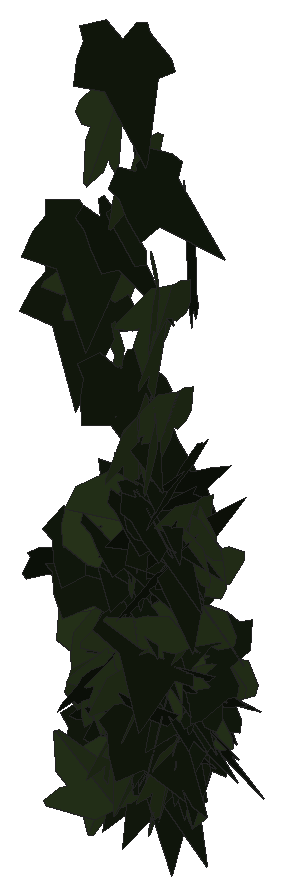
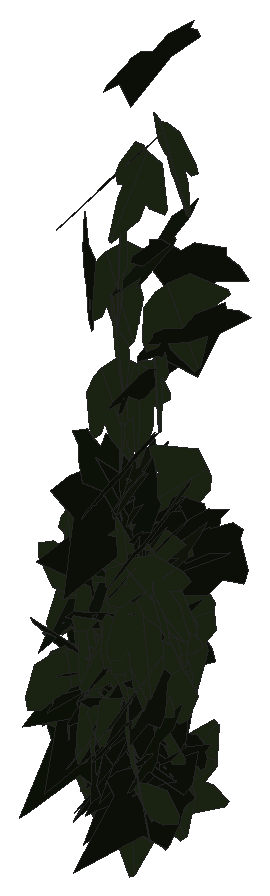
# SketchUp Ruby script. Lengths in inches.
U = 1.inch
M = Sketchup.active_model
def pt(a) = Geom::Point3d.new(a.map { |v| v * U })
def face(e, loops, mat)
  f = e.add_face(loops[0].map { |a| pt(a) })
  loops[1..].each { |l| e.add_face(l.map { |a| pt(a) }).erase! }
  f.material = f.back_material = mat if mat
  f
end
# faces: each face lists its corners as indices into pts; further lists are holes
def faces(e, pts, list, mat = nil) = list.each { |f| face(e, (f[0].is_a?(Array) ? f : [f]).map { |l| l.map { |i| pts[i] } }, mat) }
# xy, xz, yz: faces in a plane at the given z, y or x. An outline is a flat list of corners, or four numbers for a rectangle; further outlines are holes
def ring(l) = l.size == 4 ? [[l[0], l[1]], [l[2], l[1]], [l[2], l[3]], [l[0], l[3]]] : l.each_slice(2).to_a
def flat(e, list, mat, &to3) = list.each { |f| face(e, (f[0].is_a?(Array) ? f : [f]).map { |l| ring(l).map { |u, v| to3.(u, v) } }, mat) }
def xy(e, z, list, mat = nil) = flat(e, list, mat) { |x, y| [x, y, z] }
def xz(e, y, list, mat = nil) = flat(e, list, mat) { |x, z| [x, y, z] }
def yz(e, x, list, mat = nil) = flat(e, list, mat) { |y, z| [x, y, z] }
def lines(e, pts, list) = list.each { |a, b| e.add_line(pt(pts[a]), pt(pts[b])) }
# prism: a flat outline (further loops are holes) pulled along v
def prism(e, loops, v, mat = nil)
  f = face(e, loops, mat); d = Geom::Vector3d.new(v.map { |x| x * U })
  f.pushpull(f.normal.samedirection?(d) ? d.length : -d.length)
end
def box(e, o, s, mat = nil) = prism(e, [[o, [o[0] + s[0], o[1], o[2]], [o[0] + s[0], o[1] + s[1], o[2]], [o[0], o[1] + s[1], o[2]]]], [0, 0, s[2]], mat)
def at(x, y, z, deg = 0) = Geom::Transformation.translation(pt([x, y, z])) * Geom::Transformation.rotation(ORIGIN, Z_AXIS, deg.degrees)
def axes(o, x, y, z) = Geom::Transformation.new([*x, 0, *y, 0, *z, 0, *pt(o).to_a, 1])
def part(name) = M.definitions.add(name)
# library, detail: a bought-in or finely detailed component or shape, given as its bounding box
def library(name, o, s) = part(name).tap { |d| box(d.entities, o, s) }
def detail(e, o, s) = box(e.add_group.entities, o, s)
def put(e, d, t, mat = nil) = e.add_instance(d, t).tap { |i| i.material = mat if mat }
def group(e, t, mat = nil) = e.add_group.tap { |g| g.transformation = t; g.material = mat if mat }.entities
root = M.entities
M.materials.add("efeu1").color = [18, 25, 13]
M.materials.add("efeu2").color = [43, 57, 29]
c1 = part("ivyleaf_9")
p = [[1.54,2.16,1.25],[1.36,2.04,1.19],[-0.21,0.99,0.68],[-0.71,1.11,0.82],[-0.85,0.86,0.67],[-0.8,0.17,0.21],
  [-0.9,-0.01,0.1],[-0.67,-0.16,-0.02],[-0.08,-0.08,-0.05],[-0.03,-0.6,-0.4],[0.65,-0.88,-0.66],[0.83,-0.6,-0.49],
  [1.29,-0.42,-0.43],[1.8125,-0.07,-0.26],[1.21,0.44,0.15]]
faces(c1.entities,p,[[0,1,2,3,4,5,6,7,8,9,10,11,12,13,14]],"efeu1")
c2 = part("ivyleaf_10")
p = [[0,0.5,-0.03],[-0.0625,2.02,-0.43],[-0.19,2.01,-0.46],[-0.54,1.05,-0.29],[-0.52,0.625,-0.18],[-0.83,0.76,-0.28],
  [-1.16,0.64,-0.33],[-1.15,0.33,-0.24],[-0.77,-0.39,0.02],[-0.3,-0.51,0.16],[0.04,-0.48,0.23],[-0.02,2.01,-0.4375],
  [-0.06,2.01,-0.43],[0.04,-0.49,0.23],[0.67,-0.49,0.14],[1.38,0.36,-0.2],[1.375,0.51,-0.24],[0.81,0.65,-0.19],
  [0.62,0.59,-0.15],[0.6,1.09,-0.28],[0.5,1.23,-0.31]]
faces(c2.entities,p,[[0,1,2,3,4,5,6,7,8,9,10],[11,12,0,13,14,15,16,17,18,19,20]],"efeu2")
put(root,c1,axes([26.44,224.45,223.17],[0.03434,-0.04031,-0.49719],[-0.1235,0.48216,-0.04762],[0.48329,0.12607,0.02316]))
put(root,c1,axes([26.43,223.89,229.43],[-0.1338,-0.47834,-0.05732],[0.01192,0.05618,-0.49669],[0.48162,-0.13429,-0.00363]))
put(root,c2,axes([26.76,223.75,222.81],[-0.39948,-0.12303,-0.27437],[-0.26267,-0.07927,0.418],[-0.14635,0.4781,-0.0013]))
put(root,c2,axes([26.52,224.05,225.74],[0.42251,-0.26699,-0.01411],[0.00965,0.04159,-0.49817],[0.26719,0.4207,0.04029]))
put(root,c2,axes([26.54,223.99,224.24],[-0.01614,0.49352,0.0786],[-0.04607,0.07684,-0.49191],[-0.49761,-0.02312,0.043]))
put(root,c2,axes([26.63,223.85,229.71],[-0.19206,-0.43193,0.16293],[0.00554,-0.17861,-0.46698],[0.46161,-0.17758,0.07339]))
put(root,c1,axes([26.56,223.29,226.24],[0.27932,0.41465,0.00673],[0.00209,0.0067,-0.49995],[-0.4147,0.27932,0.00201]))
put(root,c2,axes([26.61,224.41,223.15],[-0.13819,-0.44837,0.17282],[0.05241,-0.19281,-0.45834],[0.47766,-0.10856,0.10029]))
put(root,c2,axes([26.65,224.33,225.1875],[-0.2081,-0.45414,-0.02115],[0.00739,0.01988,-0.49955],[0.45458,-0.20823,-0.00156]))
put(root,c2,axes([26.74,224.43,226.05],[0.41072,0.07979,-0.27376],[-0.27485,-0.0171,-0.41733],[-0.07596,0.4933,0.02982]))
put(root,c2,axes([26.6875,224.09,223.14],[-0.21542,-0.41319,0.18129],[-0.00498,-0.1987,-0.4588],[0.45119,-0.19947,0.08149]))
put(root,c2,axes([26.68,224.39,225.45],[-0.19849,-0.45883,0.00855],[-0.00252,-0.00822,-0.49993],[0.45891,-0.1985,0.00096]))
put(root,c1,axes([26.4,224.33,223.52],[0.07246,-0.41609,-0.26762],[0.06317,0.27604,-0.41208],[0.49067,0.0259,0.09257]))
put(root,c1,axes([26.5,224.11,223.78],[0.32795,0.33396,0.17584],[0.13474,0.114,-0.46781],[-0.35256,0.35422,-0.01523]))
put(root,c1,axes([26.58,224.34,223.65],[0.06737,-0.13954,-0.47538],[-0.17347,0.44275,-0.15454],[0.46408,0.18575,0.01124]))
put(root,c2,axes([26.4375,223.66,225.22],[0.07521,-0.12057,-0.47938],[0.33159,0.37192,-0.04152],[0.3666,-0.31167,0.1359]))
put(root,c1,axes([26.35,224.53,223.87],[0.27119,-0.37778,0.18368],[0.09446,-0.15819,-0.46481],[0.40931,0.28681,-0.01443]))
put(root,c2,axes([26.73,224.52,223.01],[-0.21568,-0.4492,-0.0412],[0.013,0.03945,-0.49827],[0.4509,-0.21601,-0.00534]))
put(root,c2,axes([26.34,224.25,224.72],[0.31218,-0.02984,0.38943],[0.38228,0.1255,-0.29683],[-0.08002,0.48307,0.10117]))
put(root,c1,axes([26.6,223.73,230.37],[-0.29291,-0.33308,-0.23078],[0.16591,0.16122,-0.44326],[0.3697,-0.33625,0.01608]))
put(root,c2,axes([26.74,224.38,223.43],[0.21037,-0.44106,-0.10589],[-0.02841,0.10368,-0.48831],[0.4527,0.21147,0.01857]))
put(root,c2,axes([26.68,223.42,224.73],[-0.01987,-0.09469,-0.49055],[0.09576,0.48111,-0.09675],[0.49034,-0.09779,-0.00098]))
put(root,c2,axes([26.59,224.68,223.13],[0.45407,0.1891,0.0898],[0.08226,0.03605,-0.49187],[-0.1925,0.46146,0.00163]))
put(root,c1,axes([26.68,224.32,224.57],[0.44332,0.01828,-0.2305],[-0.2311,0.05105,-0.44044],[0.00743,0.49705,0.05371]))
put(root,c1,axes([26.55,224.58,224.6875],[0.31341,-0.35026,-0.17057],[-0.08987,0.14801,-0.46906],[0.37908,0.32467,0.02981]))
put(root,c2,axes([26.88,224.06,224.34],[-0.46166,0.15733,0.11009],[-0.12274,-0.02135,-0.48423],[-0.14766,-0.47412,0.05834]))
put(root,c2,axes([26.86,224.26,223.71],[-0.4915,-0.06792,0.06174],[-0.05056,-0.08032,-0.49091],[0.0766,-0.48881,0.07209]))
put(root,c2,axes([26.76,224.43,223.94],[0.1741,-0.46161,0.0813],[0.04429,-0.07013,-0.49307],[0.46661,0.17889,0.01647]))
put(root,c2,axes([26.89,224.36,224.1875],[-0.26481,-0.4016,0.13634],[-0.03925,-0.13684,-0.47931],[0.4223,-0.26456,0.04095]))
put(root,c1,axes([26.54,223.79,225.99],[0.14825,-0.37496,-0.29568],[0.0716,0.32356,-0.37441],[0.47212,0.06867,0.14963]))
put(root,c2,axes([26.83,223.7,231.91],[0.41956,-0.24987,-0.1074],[-0.07499,0.08351,-0.48724],[0.26143,0.42496,0.0326]))
put(root,c1,axes([26.61,223.68,226.52],[0.12774,-0.33855,-0.34506],[0.00542,0.35789,-0.34912],[0.48338,0.08545,0.0951]))
put(root,c1,axes([26.63,224.2,225.99],[-0.05333,-0.39349,0.30384],[0.14531,-0.30458,-0.36894],[0.47544,0.04894,0.14684]))
put(root,c1,axes([27.02,223.44,224.77],[-0.07532,0.49266,-0.04013],[0.01024,-0.03903,-0.49837],[-0.49419,-0.0759,-0.00421]))
put(root,c2,axes([26.57,224.3125,225.77],[0.25772,-0.13671,0.40606],[0.37585,-0.15538,-0.29086],[0.20571,0.45516,0.02267]))
put(root,c1,axes([26.67,224.38,226.54],[0.10894,-0.47795,0.09847],[0.00474,-0.09986,-0.4899],[0.48796,0.10768,-0.01723]))
put(root,c1,axes([26.78,224,224.1875],[0.44004,0.23739,0.00302],[0.0022,0.00228,-0.49999],[-0.2374,0.44005,0.00096]))
put(root,c2,axes([26.98,223.81,223.73],[0.08358,-0.48207,-0.10307],[-0.02313,0.10059,-0.48923],[0.49242,0.08655,-0.00549]))
put(root,c2,axes([27.02,224.16,224.82],[-0.40766,-0.28852,0.02391],[-0.02215,-0.0101,-0.49941],[0.28866,-0.40823,-0.00455]))
put(root,c1,axes([27.04,224.625,223.44],[-0.46124,-0.18116,-0.06663],[0.06515,0.01635,-0.49547],[0.18169,-0.46574,0.00852]))
put(root,c2,axes([26.96,224.375,224.87],[0.24138,0.40825,-0.15834],[-0.14018,-0.09925,-0.46957],[-0.41483,0.27108,0.06655]))
put(root,c2,axes([27,224.19,226.3],[-0.34461,-0.35285,0.08211],[0.0193,-0.13104,-0.48214],[0.36176,-0.32913,0.10393]))
put(root,c2,axes([26.98,223.96,226.13],[0.38273,-0.3199,-0.03438],[-0.02418,0.02468,-0.4988],[0.32083,0.38348,0.00343]))
put(root,c2,axes([27.02,224.44,225.27],[0.05145,-0.49577,-0.03954],[-0.00196,0.03955,-0.49843],[0.49734,0.05144,0.00213]))
put(root,c1,axes([26.77,224.4,224],[0.17569,-0.45048,-0.12729],[-0.01864,0.12912,-0.48268],[0.46775,0.17435,0.02857]))
put(root,c2,axes([27.07,224.02,225.64],[-0.4982,-0.00904,0.0414],[-0.04139,-0.00124,-0.49828],[0.00911,-0.49992,0.00049]))
put(root,c2,axes([27.07,223.625,228.82],[0.28842,-0.32666,-0.24517],[-0.0777,0.25077,-0.42553],[0.40097,0.28356,0.09389]))
put(root,c1,axes([26.8,223.96,224.32],[0.33193,-0.33233,-0.1714],[-0.08264,0.15832,-0.46702],[0.36468,0.33836,0.05018]))
put(root,c2,axes([27.08,224.54,223.96],[-0.26496,-0.39134,0.16324],[0.00892,-0.19759,-0.45921],[0.42393,-0.24043,0.11169]))
put(root,c2,axes([27.12,223.68,224.74],[-0.15605,-0.46271,0.10748],[-0.02296,-0.10565,-0.48817],[0.47447,-0.15729,0.01172]))
put(root,c1,axes([26.79,223.71,230.51],[0.34851,-0.3414,-0.10948],[-0.03111,0.1233,-0.48356],[0.35717,0.34387,0.0647]))
put(root,c1,axes([26.83,224.0625,226.14],[0.14404,-0.47688,-0.04283],[0.00905,0.04743,-0.49766],[0.47872,0.14259,0.0223]))
put(root,c1,axes([26.89,224.38,224.97],[0.02839,-0.49889,0.01741],[-0.01213,-0.01813,-0.49952],[0.49905,0.02795,-0.01313]))
put(root,c2,axes([26.92,223.21,226.85],[0.05602,0.17558,0.46479],[0.10307,0.45346,-0.18372],[-0.48604,0.1164,0.01461]))
put(root,c1,axes([26.99,223.96,224.48],[0.44339,0.20039,-0.1151],[-0.10176,-0.05429,-0.48652],[-0.20749,0.45486,-0.00736]))
put(root,c1,axes([26.87,223.59,226.61],[0.38792,-0.27185,-0.16006],[-0.08647,0.15236,-0.46831],[0.30339,0.39101,0.07119]))
put(root,c1,axes([27.06,224.55,224.27],[-0.21472,-0.45133,-0.01395],[0.00642,0.01239,-0.49981],[0.4515,-0.21482,0.00048]))
put(root,c2,axes([27.15,224.61,223.36],[0.43176,-0.24957,-0.03598],[-0.03407,0.01295,-0.49867],[0.24984,0.43307,-0.00582]))
put(root,c2,axes([27.27,224.3,225.64],[-0.28523,-0.39451,0.11402],[-0.04605,-0.10723,-0.48619],[0.40807,-0.28786,0.02483]))
put(root,c2,axes([27.25,224.55,224.06],[-0.00998,-0.49542,-0.06681],[-0.0039,0.0669,-0.49549],[0.49989,-0.00937,-0.0052]))
put(root,c2,axes([27.24,224.34,223.09],[0.26581,-0.41937,-0.05893],[-0.03754,0.04597,-0.49646],[0.42182,0.26836,-0.00705]))
put(root,c1,axes([26.88,224.24,226.57],[0.14378,-0.22985,0.42012],[0.19859,-0.37053,-0.27069],[0.43577,0.2447,-0.01525]))
put(root,c2,axes([27.28,224.12,224.57],[0.45788,-0.13224,-0.15118],[-0.13674,0.07045,-0.47575],[0.14713,0.47702,0.02835]))
put(root,c2,axes([27.21,223.875,224.18],[0.25004,-0.42993,0.05133],[0.02402,-0.04541,-0.49735],[0.43232,0.25119,-0.00206]))
put(root,c1,axes([27.23,224.5,223.45],[-0.42778,-0.20196,-0.16191],[0.18966,-0.03172,-0.46154],[0.17616,-0.4563,0.10375]))
put(root,c1,axes([27.59,223.96,223.7],[-0.29372,0.28428,0.28795],[-0.22787,0.17782,-0.40799],[-0.33437,-0.3709,0.0251]))
put(root,c1,axes([27.36,224.0625,223.48],[-0.00091,0.35489,0.35221],[0.00044,0.35221,-0.35489],[-0.5,-0.00034,-0.00095]))
put(root,c2,axes([27.26,223.69,231.3125],[-0.04835,-0.31821,-0.38263],[0.03359,0.38147,-0.32149],[0.49652,-0.0568,-0.01551]))
put(root,c1,axes([27.03,223.71,228.5625],[0.14171,-0.45534,-0.15029],[-0.00942,0.15404,-0.47559],[0.4794,0.13763,0.03508]))
put(root,c1,axes([27.53,224.46,225.15],[-0.4353,-0.03977,0.24275],[-0.20954,-0.19852,-0.40827],[0.12886,-0.45717,0.15616]))
put(root,c1,axes([27.11,223.67,233.02],[0.05783,-0.48465,-0.10847],[-0.00618,0.10849,-0.48805],[0.49661,0.05779,0.00656]))
put(root,c2,axes([27.31,223.85,223.75],[0.03723,-0.45282,0.20874],[0.03434,-0.20649,-0.45407],[0.49743,0.04815,0.01573]))
put(root,c1,axes([27.1,224.48,223.11],[0.08167,-0.48734,0.07635],[-0.00105,-0.07757,-0.49395],[0.49328,0.08052,-0.0137]))
put(root,c1,axes([27.45,223.77,226.75],[-0.0152,0.48939,-0.10134],[-0.009,-0.10163,-0.48948],[-0.49969,-0.01306,0.0119]))
put(root,c2,axes([27.64,224.17,223.01],[0.06685,0.10187,-0.48492],[-0.43373,0.24864,-0.00756],[0.2396,0.42166,0.12162]))
put(root,c1,axes([27.05,223.6,224.09],[0.47297,0.11596,0.11337],[0.10644,0.04177,-0.48675],[-0.12236,0.48457,0.01482]))
put(root,c2,axes([27.32,224.2,224.375],[-0.07901,-0.49106,-0.05114],[0.05821,0.04217,-0.49481],[0.49028,-0.08414,0.0505]))
put(root,c1,axes([27.08,224.42,223.24],[0.21723,-0.44191,-0.08675],[-0.01866,0.0874,-0.49195],[0.44996,0.21697,0.02148]))
put(root,c1,axes([27.09,224.31,227.37],[0.151,-0.47598,0.02538],[0.00375,-0.02544,-0.49934],[0.47664,0.15099,-0.00411]))
put(root,c1,axes([27.54,224.02,226.19],[-0.26772,0.41814,-0.05906],[0.02682,-0.05294,-0.49646],[-0.42144,-0.26899,0.00592]))
put(root,c1,axes([27.31,224.12,226.79],[0.19154,0.43859,0.14476],[0.07527,0.12498,-0.47824],[-0.45568,0.205,-0.01815]))
put(root,c2,axes([27.52,224.35,226],[-0.4159,-0.16799,0.22092],[-0.18339,-0.13238,-0.44592],[0.20831,-0.45194,0.0485]))
put(root,c2,axes([27.18,223.98,224.81],[0.41853,0.23581,0.13865],[0.10577,0.09422,-0.47952],[-0.25228,0.43072,0.02898]))
put(root,c2,axes([27.29,224.17,224.09],[0.33216,-0.36097,0.09681],[0.07293,-0.06443,-0.49044],[0.36654,0.33993,0.00985]))
put(root,c2,axes([27.54,224.16,226.35],[-0.45422,0.09333,0.18702],[-0.19547,-0.03124,-0.45915],[-0.07402,-0.49022,0.06487]))
put(root,c2,axes([27.42,223.55,225.32],[-0.40994,-0.28399,-0.03601],[0.03691,0.00994,-0.49854],[0.28388,-0.4114,0.01282]))
put(root,c2,axes([27.4,223.52,224.78],[-0.16454,-0.42564,-0.20435],[0.05693,0.19694,-0.45604],[0.46871,-0.17334,-0.01634]))
put(root,c1,axes([27.3,224.39,224.22],[0.44246,0.21869,-0.08005],[-0.08916,0.0003,-0.49199],[-0.21514,0.44964,0.03926]))
put(root,c1,axes([27.1875,223.68,226.9],[0.39758,-0.27644,-0.12452],[-0.06426,0.12384,-0.48014],[0.2963,0.3978,0.06295]))
put(root,c2,axes([27.46,223.45,228.1],[0.09785,-0.46193,-0.16446],[0.0063,0.16888,-0.47057],[0.49029,0.09002,0.03887]))
put(root,c1,axes([27.64,223.73,226.11],[-0.21588,0.43126,-0.13196],[0.0405,-0.12717,-0.48186],[-0.44917,-0.21873,0.01997]))
put(root,c2,axes([27.48,224.42,223.88],[-0.49964,-0.01625,-0.00989],[0.01317,-0.10778,-0.48807],[0.01373,-0.48797,0.10813]))
put(root,c1,axes([27.23,224.5,223.82],[0.1064,-0.46848,0.13859],[0.02728,-0.13592,-0.4804],[0.48779,0.10979,-0.00336]))
put(root,c2,axes([27.43,224.125,224.45],[-0.4894,-0.01059,-0.10188],[0.10162,0.0121,-0.48941],[0.01283,-0.49974,-0.0097]))
put(root,c1,axes([27.2,224.32,224.76],[0.28265,-0.41237,0.0079],[0.02224,0.00567,-0.49947],[0.41184,0.2827,0.02155]))
put(root,c1,axes([27.22,224.1,224.47],[0.47572,0.09088,0.12424],[0.09862,0.1299,-0.47265],[-0.11818,0.4742,0.10566]))
put(root,c2,axes([27.5,224.25,226.5],[-0.4871,0.11065,-0.02214],[0.02237,-0.00146,-0.4995],[-0.1106,-0.4876,-0.00353]))
put(root,c1,axes([27.72,223.9,227.24],[-0.25718,0.42855,0.01409],[-0.00448,0.01374,-0.49979],[-0.42876,-0.2572,-0.00322]))
put(root,c1,axes([27.51,224.38,224.43],[-0.33268,-0.35757,0.10712],[0.01506,-0.15622,-0.47473],[0.37296,-0.31264,0.11471]))
put(root,c2,axes([27.53,223.83,229.2],[0.19892,-0.44311,-0.11867],[-0.01432,0.12328,-0.48435],[0.4585,0.1961,0.03636]))
put(root,c2,axes([27.56,224.39,223.6875],[0.02674,-0.48712,0.10952],[-0.00049,-0.1097,-0.48782],[0.49928,0.02598,-0.00634]))
put(root,c2,axes([27.55,224.35,224.83],[0.11596,-0.47645,-0.09771],[-0.00286,0.09978,-0.48993],[0.48636,0.11419,0.02042]))
put(root,c1,axes([27.33,223.71,226.97],[0.40763,-0.20507,-0.2044],[-0.11315,0.21209,-0.43842],[0.26652,0.40369,0.1265]))
put(root,c2,axes([27.59,223.93,228.21],[-0.01148,-0.48749,0.11056],[0.00841,-0.11077,-0.4875],[0.4998,-0.00934,0.01074]))
put(root,c2,axes([27.57,224.45,225.8],[-0.39508,-0.30526,-0.02701],[-0.02299,-0.01442,0.49926],[-0.30559,0.39574,-0.00264]))
put(root,c1,axes([27.49,223.96,225.96],[0.06957,0.12894,0.47805],[0.24492,0.41059,-0.14638],[-0.43032,0.25454,-0.00603]))
put(root,c1,axes([27.375,223.86,225.13],[-0.04772,-0.46089,0.1879],[0.08863,-0.19361,-0.45239],[0.48976,-0.00986,0.10018]))
put(root,c1,axes([27.39,224.17,224.23],[0.41257,-0.20883,-0.19019],[-0.14384,0.13442,-0.45961],[0.24309,0.43396,0.05084]))
put(root,c1,axes([27.3,223.99,226.85],[0.24124,-0.43752,-0.01963],[0.02424,0.03572,-0.49813],[0.43728,0.23938,0.03844]))
put(root,c2,axes([27.6,223.6,228.02],[0.24919,-0.36679,-0.23102],[-0.0256,0.25356,-0.43018],[0.43273,0.22621,0.10759]))
put(root,c2,axes([27.69,224.19,225.3],[-0.39933,-0.28537,0.0954],[-0.05662,-0.08444,-0.48956],[0.29552,-0.40179,0.03513]))
put(root,c1,axes([27.41,224.57,223.74],[0.48429,-0.04355,-0.11647],[-0.11312,0.04014,-0.48538],[0.05163,0.49648,0.02902]))
put(root,c2,axes([27.62,223.89,223.57],[0.1196,-0.4834,-0.04493],[0.00117,0.04656,-0.49783],[0.48548,0.11898,0.01227]))
put(root,c2,axes([27.67,224.18,226.67],[-0.02871,-0.49375,0.07336],[-0.01685,-0.07249,-0.49443],[0.49889,-0.03086,-0.01248]))
put(root,c1,axes([27.52,224.51,224.21],[-0.11314,-0.48675,0.01646],[-0.00461,-0.01583,-0.49973],[0.48701,-0.11323,-0.00091]))
put(root,c1,axes([27.41,223.625,224.17],[0.18975,-0.37434,-0.27178],[-0.03556,0.28108,-0.41198],[0.46123,0.17568,0.08005]))
put(root,c2,axes([27.67,223.75,229.75],[-0.04663,-0.48942,0.09106],[0.00712,-0.0921,-0.49139],[0.49777,-0.04454,0.01556]))
put(root,c1,axes([27.4,224.57,223.64],[0.08489,-0.44341,0.2149],[0.04599,-0.20999,-0.45143],[0.49059,0.09641,0.00513]))
put(root,c2,axes([27.69,223.53,230],[0.23363,-0.32317,-0.30162],[-0.06721,0.31122,-0.38552],[0.43692,0.22068,0.10198]))
put(root,c2,axes([27.7,224.32,224.4375],[-0.37217,-0.33318,0.02199],[-0.00464,-0.02777,-0.49921],[0.33387,-0.37178,0.01758]))
put(root,c1,axes([27.81,224.09,229.68],[0.02328,-0.08856,0.49154],[-0.0851,0.48418,0.09127],[-0.49215,-0.08791,0.00746]))
put(root,c2,axes([27.72,224.58,224.43],[-0.34535,-0.35208,0.08231],[-0.02416,-0.0911,-0.49104],[0.36077,-0.34313,0.04591]))
put(root,c1,axes([27.42,223.61,231.41],[0.32499,-0.28394,-0.2525],[-0.06839,0.28312,-0.4064],[0.37377,0.29869,0.14519]))
put(root,c1,axes([27.47,224.21,226.4],[0.05792,-0.49374,-0.05355],[-0.00054,0.05385,-0.49709],[0.49663,0.05764,0.0057]))
put(root,c1,axes([28.05,224.41,224.69],[-0.40449,0.20954,0.20611],[-0.22052,0.01546,-0.44848],[-0.19432,-0.45371,0.07991]))
put(root,c1,axes([27.53,224.21,225.87],[0.45739,-0.1376,-0.14786],[-0.14189,0.04162,-0.47764],[0.14375,0.47889,-0.00097]))
